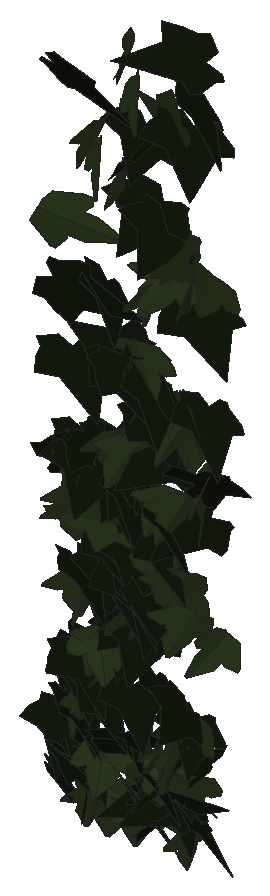
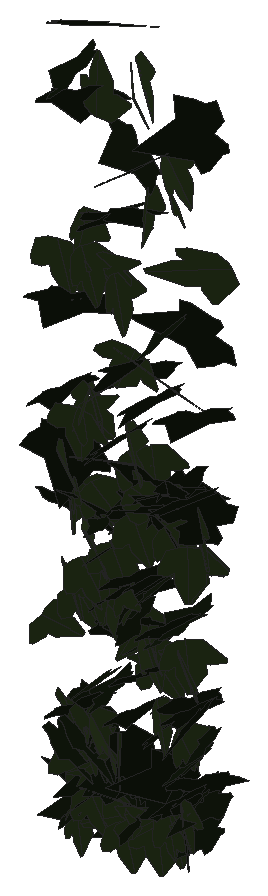
# SketchUp Ruby script. Lengths in inches.
U = 1.inch
M = Sketchup.active_model
def pt(a) = Geom::Point3d.new(a.map { |v| v * U })
def face(e, loops, mat)
  f = e.add_face(loops[0].map { |a| pt(a) })
  loops[1..].each { |l| e.add_face(l.map { |a| pt(a) }).erase! }
  f.material = f.back_material = mat if mat
  f
end
# faces: each face lists its corners as indices into pts; further lists are holes
def faces(e, pts, list, mat = nil) = list.each { |f| face(e, (f[0].is_a?(Array) ? f : [f]).map { |l| l.map { |i| pts[i] } }, mat) }
# xy, xz, yz: faces in a plane at the given z, y or x. An outline is a flat list of corners, or four numbers for a rectangle; further outlines are holes
def ring(l) = l.size == 4 ? [[l[0], l[1]], [l[2], l[1]], [l[2], l[3]], [l[0], l[3]]] : l.each_slice(2).to_a
def flat(e, list, mat, &to3) = list.each { |f| face(e, (f[0].is_a?(Array) ? f : [f]).map { |l| ring(l).map { |u, v| to3.(u, v) } }, mat) }
def xy(e, z, list, mat = nil) = flat(e, list, mat) { |x, y| [x, y, z] }
def xz(e, y, list, mat = nil) = flat(e, list, mat) { |x, z| [x, y, z] }
def yz(e, x, list, mat = nil) = flat(e, list, mat) { |y, z| [x, y, z] }
def lines(e, pts, list) = list.each { |a, b| e.add_line(pt(pts[a]), pt(pts[b])) }
# prism: a flat outline (further loops are holes) pulled along v
def prism(e, loops, v, mat = nil)
  f = face(e, loops, mat); d = Geom::Vector3d.new(v.map { |x| x * U })
  f.pushpull(f.normal.samedirection?(d) ? d.length : -d.length)
end
def box(e, o, s, mat = nil) = prism(e, [[o, [o[0] + s[0], o[1], o[2]], [o[0] + s[0], o[1] + s[1], o[2]], [o[0], o[1] + s[1], o[2]]]], [0, 0, s[2]], mat)
def at(x, y, z, deg = 0) = Geom::Transformation.translation(pt([x, y, z])) * Geom::Transformation.rotation(ORIGIN, Z_AXIS, deg.degrees)
def axes(o, x, y, z) = Geom::Transformation.new([*x, 0, *y, 0, *z, 0, *pt(o).to_a, 1])
def part(name) = M.definitions.add(name)
# library, detail: a bought-in or finely detailed component or shape, given as its bounding box
def library(name, o, s) = part(name).tap { |d| box(d.entities, o, s) }
def detail(e, o, s) = box(e.add_group.entities, o, s)
def put(e, d, t, mat = nil) = e.add_instance(d, t).tap { |i| i.material = mat if mat }
def group(e, t, mat = nil) = e.add_group.tap { |g| g.transformation = t; g.material = mat if mat }.entities
root = M.entities
M.materials.add("1026 AP 7946 SUNNY SIDE UP").color = [254, 231, 186]
M.materials.add("efeu1").color = [18, 25, 13]
M.materials.add("efeu2").color = [43, 57, 29]
c1 = part("ivyleaf_10")
p = [[0,0.5,-0.03],[-0.0625,2.02,-0.43],[-0.19,2.01,-0.46],[-0.54,1.05,-0.29],[-0.52,0.625,-0.18],[-0.83,0.76,-0.28],
  [-1.16,0.64,-0.33],[-1.15,0.33,-0.24],[-0.77,-0.39,0.02],[-0.3,-0.51,0.16],[0.04,-0.48,0.23],[-0.02,2.01,-0.4375],
  [-0.06,2.01,-0.43],[0.04,-0.49,0.23],[0.67,-0.49,0.14],[1.38,0.36,-0.2],[1.375,0.51,-0.24],[0.81,0.65,-0.19],
  [0.62,0.59,-0.15],[0.6,1.09,-0.28],[0.5,1.23,-0.31]]
faces(c1.entities,p,[[0,1,2,3,4,5,6,7,8,9,10],[11,12,0,13,14,15,16,17,18,19,20]],"efeu2")
c2 = part("ivyleaf_9")
p = [[1.54,2.16,1.25],[1.36,2.04,1.19],[-0.21,0.99,0.68],[-0.71,1.11,0.82],[-0.85,0.86,0.67],[-0.8,0.17,0.21],
  [-0.9,-0.01,0.1],[-0.67,-0.16,-0.02],[-0.08,-0.08,-0.05],[-0.03,-0.6,-0.4],[0.65,-0.88,-0.66],[0.83,-0.6,-0.49],
  [1.29,-0.42,-0.43],[1.8125,-0.07,-0.26],[1.21,0.44,0.15]]
faces(c2.entities,p,[[0,1,2,3,4,5,6,7,8,9,10,11,12,13,14]],"efeu1")
put(root,c1,axes([111.16,212.79,270.9],[-0.25846,-0.22574,0.01408],[0.03079,-0.0326,-0.2856],[0.3544,-0.1618,0.03508]),"1026 AP 7946 SUNNY SIDE UP")
put(root,c2,axes([111.02,212.73,270.01],[0.18307,-0.18563,-0.16634],[-0.13918,0.13382,-0.22493],[0.35979,0.14622,-0.00237]),"1026 AP 7946 SUNNY SIDE UP")
put(root,c2,axes([111.1,212.61,268.95],[-0.21823,-0.23774,-0.01451],[0.02596,0.00509,-0.28331],[0.37346,-0.13928,0.01122]),"1026 AP 7946 SUNNY SIDE UP")
put(root,c2,axes([111.03,212.36,268.65],[0.37718,-0.03348,-0.11398],[-0.14053,0.1073,-0.23284],[0.11482,0.2413,0.08945]),"1026 AP 7946 SUNNY SIDE UP")
put(root,c1,axes([111.21,212.71,272.2],[-0.28974,-0.20895,-0.01101],[0.02661,-0.00228,-0.28664],[0.32781,-0.18449,0.01354]),"1026 AP 7946 SUNNY SIDE UP")
put(root,c1,axes([111.15,212.85,270.75],[0.24057,-0.22294,0.04507],[0.03997,-0.03716,-0.27877],[0.35539,0.15509,0.00084]),"1026 AP 7946 SUNNY SIDE UP")
put(root,c2,axes([111.01,212.41,268.2],[0.32875,-0.14193,-0.07795],[-0.07623,0.06134,-0.25893],[0.24052,0.21343,0.02448]),"1026 AP 7946 SUNNY SIDE UP")
put(root,c1,axes([111.29,212.4375,272.7],[0.23704,-0.24789,-0.14116],[-0.07303,0.12988,-0.297],[0.43826,0.15572,0.02686]),"1026 AP 7946 SUNNY SIDE UP")
put(root,c1,axes([111.28,212.54,272.11],[-0.21849,-0.24101,-0.02736],[0.02828,0.0187,-0.28642],[0.37998,-0.13997,0.00559]),"1026 AP 7946 SUNNY SIDE UP")
put(root,c2,axes([110.98,212.5,272.71],[0.11914,0.00468,0.28145],[0.4221,0.05149,-0.07731],[-0.07996,0.27878,0.01124]),"1026 AP 7946 SUNNY SIDE UP")
put(root,c2,axes([111.15,212.62,274.31],[-0.07232,-0.26894,-0.11603],[0.07636,0.10381,-0.27897],[0.45113,-0.06068,0.02862]),"1026 AP 7946 SUNNY SIDE UP")
put(root,c2,axes([111.17,212.73,269.19],[0.05394,-0.25714,0.06466],[0.01516,-0.0635,-0.26762],[0.41647,0.03561,0.00137]),"1026 AP 7946 SUNNY SIDE UP")
put(root,c2,axes([111,212.51,278.44],[0.46882,-0.09984,0.08402],[0.11016,-0.04873,-0.32333],[0.17085,0.3054,-0.02209]),"1026 AP 7946 SUNNY SIDE UP")
put(root,c2,axes([111.16,212.46,269.32],[0.20675,-0.23514,0.01184],[-0.00657,-0.01702,-0.27737],[0.37023,0.13101,-0.01153]),"1026 AP 7946 SUNNY SIDE UP")
put(root,c1,axes([111.04,212.39,276.37],[-0.14408,-0.08172,-0.31235],[0.478,0.0542,-0.10955],[0.12093,-0.31162,0.06085]),"1026 AP 7946 SUNNY SIDE UP")
put(root,c2,axes([111.21,212.74,273.08],[0.01746,-0.27644,-0.08279],[0.03076,0.07939,-0.28366],[0.45094,0.00529,0.02255]),"1026 AP 7946 SUNNY SIDE UP")
put(root,c2,axes([111.23,212.34,268.62],[0.25425,-0.18608,-0.12792],[-0.11025,0.10197,-0.25304],[0.33307,0.1758,0.01389]),"1026 AP 7946 SUNNY SIDE UP")
put(root,c1,axes([111.41,212.79,272.52],[-0.18292,-0.21073,0.15461],[0.05122,-0.17635,-0.22829],[0.40466,-0.07293,0.09878]),"1026 AP 7946 SUNNY SIDE UP")
put(root,c1,axes([111.4375,212.57,268.41],[0.31397,-0.14487,-0.09904],[-0.06966,0.09792,-0.24836],[0.26363,0.19841,0.05232]),"1026 AP 7946 SUNNY SIDE UP")
put(root,c2,axes([111.3,212.55,269.875],[-0.02897,-0.26788,-0.02364],[0.00054,0.02146,-0.27649],[0.42255,-0.01839,-0.00127]),"1026 AP 7946 SUNNY SIDE UP")
put(root,c2,axes([111.6,212.33,268.21],[0.01774,-0.02013,-0.27651],[-0.37306,0.12588,-0.01928],[0.19948,0.2372,-0.01145]),"1026 AP 7946 SUNNY SIDE UP")
put(root,c1,axes([111.76,212.4,272.11],[0.11792,-0.02448,-0.28807],[-0.42407,0.07343,-0.08075],[0.12157,0.2799,-0.00225]),"1026 AP 7946 SUNNY SIDE UP")
put(root,c1,axes([111.44,212.51,269.39],[-0.03187,-0.24501,0.11408],[0.06089,-0.11393,-0.24991],[0.41929,-0.00208,0.04496]),"1026 AP 7946 SUNNY SIDE UP")
put(root,c2,axes([111.34,212.71,268.62],[0.01428,-0.26436,-0.03819],[-0.01447,0.03526,-0.27217],[0.41918,0.01022,-0.00809]),"1026 AP 7946 SUNNY SIDE UP")
put(root,c2,axes([111.33,212.53,270.02],[-0.01544,-0.26714,-0.10615],[0.01368,0.10126,-0.27476],[0.44916,-0.01227,0.00472]),"1026 AP 7946 SUNNY SIDE UP")
put(root,c2,axes([111.07,212.4,275.41],[0.17756,-0.03565,-0.29261],[0.36941,0.18565,0.07336],[0.25662,-0.24258,0.09686]),"1026 AP 7946 SUNNY SIDE UP")
put(root,c2,axes([111.3,212.58,271.2],[0.07275,-0.25296,0.09975],[0.07853,-0.09004,-0.26355],[0.41942,0.06074,0.03205]),"1026 AP 7946 SUNNY SIDE UP")
put(root,c2,axes([111.45,212.5,273.23],[0.09054,-0.1877,-0.21569],[-0.12355,0.19332,-0.20071],[0.42323,0.09659,-0.01245]),"1026 AP 7946 SUNNY SIDE UP")
put(root,c1,axes([111.625,212.51,268.09],[-0.15001,-0.26777,0.02721],[-0.00092,-0.02943,-0.29285],[0.42332,-0.09495,0.00901]),"1026 AP 7946 SUNNY SIDE UP")
put(root,c1,axes([111.62,212.51,277.78],[0.02832,-0.2977,0.06216],[-0.00462,-0.0623,-0.30754],[0.47813,0.01703,-0.00665]),"1026 AP 7946 SUNNY SIDE UP")
put(root,c2,axes([111.49,212.82,271.17],[-0.10353,-0.26958,0.02946],[0.00172,-0.03126,-0.28594],[0.42653,-0.06531,0.0083]),"1026 AP 7946 SUNNY SIDE UP")
put(root,c2,axes([111.58,212.53,272.95],[-0.27863,-0.23651,-0.01871],[0.02847,0.00744,-0.30423],[0.37173,-0.17784,0.00928]),"1026 AP 7946 SUNNY SIDE UP")
put(root,c1,axes([111.63,212.74,269.82],[0.03868,-0.2682,-0.04132],[0.01948,0.03982,-0.27675],[0.42562,0.02255,0.01642]),"1026 AP 7946 SUNNY SIDE UP")
put(root,c2,axes([111.46,212.9,271.85],[0.08262,-0.27136,0.03007],[-0.00016,-0.03131,-0.28486],[0.42941,0.0522,-0.00589]),"1026 AP 7946 SUNNY SIDE UP")
put(root,c1,axes([111.88,212.79,272.92],[-0.21743,-0.11557,0.22862],[-0.17064,-0.20156,-0.17845],[0.35551,-0.16743,0.05417]),"1026 AP 7946 SUNNY SIDE UP")
put(root,c1,axes([111.5625,212.58,277.39],[0.22743,-0.18145,0.19332],[0.2154,-0.13123,-0.23896],[0.35075,0.19825,0.0214]),"1026 AP 7946 SUNNY SIDE UP")
put(root,c2,axes([111.4375,212.48,268.71],[0.27503,0.06669,0.19674],[0.28969,0.0505,-0.19209],[-0.12996,0.25371,-0.01184]),"1026 AP 7946 SUNNY SIDE UP")
put(root,c1,axes([111.81,212.6,267.9],[-0.38126,-0.08092,0.04408],[-0.05632,-0.02903,-0.26299],[0.13282,-0.24458,0.01502]),"1026 AP 7946 SUNNY SIDE UP")
put(root,c2,axes([111.57,212.77,275.36],[0.04299,-0.27364,0.11977],[0.00071,-0.11827,-0.28379],[0.46845,0.02529,-0.01056]),"1026 AP 7946 SUNNY SIDE UP")
put(root,c1,axes([111.83,212.55,270.375],[-0.23292,-0.20064,0.1353],[-0.04028,-0.14155,-0.25118],[0.3759,-0.13949,0.05692]),"1026 AP 7946 SUNNY SIDE UP")
put(root,c2,axes([112.1,212.5,274.59],[-0.14094,0.20077,0.19345],[-0.27447,0.10961,-0.20718],[-0.33235,-0.17566,0.08906]),"1026 AP 7946 SUNNY SIDE UP")
put(root,c2,axes([111.62,212.53,269.56],[0.10649,-0.25155,-0.06729],[-0.02601,0.06171,-0.26801],[0.40726,0.06972,0.00048]),"1026 AP 7946 SUNNY SIDE UP")
put(root,c1,axes([111.76,212.46,268.68],[0.31294,0.17171,-0.04724],[-0.03914,-0.04271,-0.27055],[-0.2771,0.19994,-0.01514]),"1026 AP 7946 SUNNY SIDE UP")
put(root,c1,axes([111.875,212.68,270.65],[0.01039,-0.27822,0.0172],[-0.00063,-0.01829,-0.28681],[0.43842,0.00657,-0.00082]),"1026 AP 7946 SUNNY SIDE UP")
put(root,c1,axes([111.78,212.71,270.76],[0.18971,-0.23068,0.09571],[0.10543,-0.07076,-0.26736],[0.37736,0.13574,0.02658]),"1026 AP 7946 SUNNY SIDE UP")
put(root,c1,axes([111.74,212.41,270.37],[0.37299,0.1356,0.03339],[0.06446,-0.00827,-0.28012],[-0.20925,0.23917,-0.02677]),"1026 AP 7946 SUNNY SIDE UP")
put(root,c1,axes([111.92,212.52,273.36],[-0.15328,-0.26613,-0.02058],[0.01419,0.01635,-0.29187],[0.41923,-0.09786,0.00236]),"1026 AP 7946 SUNNY SIDE UP")
put(root,c1,axes([111.95,212.85,272.5],[-0.2289,-0.23113,0.07102],[-0.01115,-0.0779,-0.27962],[0.37968,-0.14163,0.03461]),"1026 AP 7946 SUNNY SIDE UP")
put(root,c2,axes([111.72,212.68,271.78],[0.02557,-0.28175,-0.04899],[0.01846,0.04665,-0.2901],[0.4485,0.01414,0.01474]),"1026 AP 7946 SUNNY SIDE UP")
put(root,c2,axes([111.9,212.87,272.74],[-0.2865,-0.21554,0.03044],[0.01372,-0.04732,-0.28853],[0.34208,-0.17862,0.03707]),"1026 AP 7946 SUNNY SIDE UP")
put(root,c2,axes([111.64,212.69,268.45],[0.0828,-0.16289,0.20919],[0.15416,-0.18052,-0.17564],[0.38042,0.10861,0.02564]),"1026 AP 7946 SUNNY SIDE UP")
put(root,c2,axes([111.87,212.92,270.37],[-0.15472,-0.24477,0.06216],[0.00463,-0.06736,-0.27073],[0.3969,-0.09463,0.02739]),"1026 AP 7946 SUNNY SIDE UP")
put(root,c2,axes([111.73,212.79,273.23],[-0.16285,-0.16476,-0.21714],[0.32064,0.09627,-0.18099],[0.27052,-0.21329,0.0838]),"1026 AP 7946 SUNNY SIDE UP")
put(root,c2,axes([111.77,212.7,274.375],[0.07629,-0.27385,-0.10286],[0.00648,0.10028,-0.28516],[0.45745,0.04425,0.02119]),"1026 AP 7946 SUNNY SIDE UP")
put(root,c2,axes([111.85,212.76,272.67],[-0.25159,-0.07127,-0.22509],[0.35615,-0.00667,-0.16899],[0.05752,-0.2704,0.0618]),"1026 AP 7946 SUNNY SIDE UP")
put(root,c1,axes([111.97,212.53,277.15],[0.07505,-0.27677,-0.10696],[0.07507,0.10947,-0.28163],[0.45784,0.02742,0.06371]),"1026 AP 7946 SUNNY SIDE UP")
put(root,c2,axes([111.98,212.84,272.81],[-0.21624,-0.24121,0.06611],[-0.01669,-0.0691,-0.28534],[0.39267,-0.13577,0.02427]),"1026 AP 7946 SUNNY SIDE UP")
put(root,c1,axes([112.05,212.6,279.05],[0.1584,-0.28964,-0.0546],[-0.01324,0.05143,-0.31549],[0.46234,0.1007,0.00968]),"1026 AP 7946 SUNNY SIDE UP")
put(root,c2,axes([111.98,212.6875,270.64],[-0.20538,-0.17712,0.17917],[0.00019,-0.19758,-0.20717],[0.39143,-0.09284,0.09411]),"1026 AP 7946 SUNNY SIDE UP")
put(root,c1,axes([112.09,212.76,273.71],[0.11088,-0.27678,-0.06673],[-0.02168,0.06171,-0.29387],[0.44588,0.07183,0.00231]),"1026 AP 7946 SUNNY SIDE UP")
put(root,c1,axes([112.16,212.59,273.24],[-0.18839,-0.21685,0.16013],[-0.035,-0.16298,-0.25089],[0.41919,-0.11106,0.05102]),"1026 AP 7946 SUNNY SIDE UP")
put(root,c1,axes([111.91,212.61,268.06],[0.15644,0.14512,0.20508],[0.15592,0.17196,-0.17995],[-0.35344,0.1401,0.01139]),"1026 AP 7946 SUNNY SIDE UP")
put(root,c2,axes([112.02,212.43,268.98],[0.30608,0.18291,0.02594],[0.05096,0.00064,-0.27426],[-0.28559,0.19615,-0.02114]),"1026 AP 7946 SUNNY SIDE UP")
put(root,c2,axes([112.04,212.98,277.7],[-0.13932,-0.26153,0.11927],[0.00228,-0.12315,-0.28253],[0.45067,-0.08023,0.0383]),"1026 AP 7946 SUNNY SIDE UP")
put(root,c1,axes([112.18,212.76,267.87],[-0.2446,-0.20952,0.03719],[0.00438,-0.0482,-0.26725],[0.3346,-0.15253,0.03069]),"1026 AP 7946 SUNNY SIDE UP")
put(root,c2,axes([112.07,212.8,271.69],[-0.13197,-0.26759,0.01194],[0.00912,-0.01555,-0.28881],[0.42117,-0.08351,0.00999]),"1026 AP 7946 SUNNY SIDE UP")
put(root,c2,axes([112.03,212.73,272.55],[-0.02936,-0.26574,0.11334],[0.01683,-0.11232,-0.27453],[0.45285,-0.01305,0.01755]),"1026 AP 7946 SUNNY SIDE UP")
put(root,c1,axes([112.16,212.39,270.87],[-0.10633,-0.21266,-0.22532],[0.14199,0.19874,-0.22793],[0.45676,-0.11129,0.01841]),"1026 AP 7946 SUNNY SIDE UP")
put(root,c2,axes([112.1,212.55,271.42],[-0.08499,-0.26836,-0.06513],[0.02002,0.06038,-0.28166],[0.43252,-0.05553,0.00024]),"1026 AP 7946 SUNNY SIDE UP")
put(root,c2,axes([112.09,212.67,269.67],[-0.03683,-0.2761,-0.01817],[0.00797,0.0157,-0.28534],[0.4348,-0.02367,0.00369]),"1026 AP 7946 SUNNY SIDE UP")
put(root,c2,axes([111.97,212.79,271.09],[0.2428,-0.21898,0.07818],[0.06371,-0.06579,-0.27639],[0.35946,0.15958,-0.00382]),"1026 AP 7946 SUNNY SIDE UP")
put(root,c2,axes([112.07,212.72,268.12],[0.28372,-0.19281,-0.00282],[-0.02004,-0.00969,-0.2716],[0.30252,0.18018,-0.01535]),"1026 AP 7946 SUNNY SIDE UP")
put(root,c1,axes([112.39,212.75,271.9],[-0.30448,-0.18758,0.08222],[-0.01057,-0.10552,-0.26935],[0.32103,-0.18139,0.06911]),"1026 AP 7946 SUNNY SIDE UP")
put(root,c2,axes([112.38,212.3,277.67],[-0.21295,0.20476,-0.20307],[-0.14326,0.17691,0.25335],[0.42467,0.16236,-0.01636]),"1026 AP 7946 SUNNY SIDE UP")
put(root,c1,axes([112.35,212.66,269.04],[0.09195,-0.25133,-0.08147],[0.03376,0.08385,-0.26241],[0.41224,0.04919,0.03966]),"1026 AP 7946 SUNNY SIDE UP")
put(root,c2,axes([112.125,212.57,271.18],[0.12771,-0.24366,0.10852],[0.04541,-0.10285,-0.26516],[0.41581,0.08607,-0.00438]),"1026 AP 7946 SUNNY SIDE UP")
put(root,c2,axes([112.12,212.45,274.61],[0.06742,-0.239,-0.19751],[0.09943,0.19501,-0.23641],[0.47004,-0.00697,0.07834]),"1026 AP 7946 SUNNY SIDE UP")
put(root,c1,axes([112.31,212.54,274.7],[-0.42802,0.04324,-0.08897],[0.10282,-0.10846,-0.26814],[-0.11224,-0.26426,0.09365]),"1026 AP 7946 SUNNY SIDE UP")
put(root,c2,axes([112.59,212.74,268.26],[-0.41159,-0.00773,0.04508],[-0.05948,-0.09892,-0.25141],[0.0368,-0.24628,0.09789]),"1026 AP 7946 SUNNY SIDE UP")
put(root,c1,axes([112.4,212.68,271],[0.02898,-0.21953,0.1827],[0.03802,-0.1771,-0.22787],[0.44336,0.02954,0.0076]),"1026 AP 7946 SUNNY SIDE UP")
put(root,c2,axes([112.2,212.77,273.71],[0.1302,-0.26337,-0.10162],[-0.01055,0.0994,-0.28292],[0.44127,0.08009,0.02322]),"1026 AP 7946 SUNNY SIDE UP")
put(root,c1,axes([112.19,212.54,278.56],[0.19897,-0.11768,0.25994],[0.27844,-0.1808,-0.17895],[0.33905,0.21754,-0.00558]),"1026 AP 7946 SUNNY SIDE UP")
put(root,c2,axes([112.47,212.74,276.87],[-0.33655,-0.20901,0.05606],[-0.01009,-0.07205,-0.30491],[0.33993,-0.20908,0.04645]),"1026 AP 7946 SUNNY SIDE UP")
put(root,c2,axes([112.42,212.54,270.75],[-0.25067,-0.22647,-0.01409],[0.02292,0.00488,-0.28513],[0.3559,-0.15983,0.00844]),"1026 AP 7946 SUNNY SIDE UP")
put(root,c1,axes([112.48,212.55,275.69],[-0.02663,-0.29967,-0.02807],[0.02088,0.02482,-0.30882],[0.47244,-0.01799,0.01206]),"1026 AP 7946 SUNNY SIDE UP")
put(root,c2,axes([112.71,212.39,268.55],[-0.19917,0.24624,0.00136],[-0.01589,-0.00528,-0.28506],[-0.38686,-0.12656,0.011]),"1026 AP 7946 SUNNY SIDE UP")
put(root,c1,axes([112.54,212.54,268.84],[0.0918,-0.26057,0.00276],[-0.00584,-0.00509,-0.27508],[0.40973,0.05831,-0.00454]),"1026 AP 7946 SUNNY SIDE UP")
put(root,c2,axes([112.63,212.8,273.21],[-0.39722,-0.11769,0.06822],[-0.01035,-0.13078,-0.26341],[0.21261,-0.22625,0.11464]),"1026 AP 7946 SUNNY SIDE UP")
put(root,c1,axes([112.57,212.65,271.33],[-0.43709,0.02439,0.00365],[-0.00896,-0.02615,-0.28632],[-0.03768,-0.27676,0.02572]),"1026 AP 7946 SUNNY SIDE UP")
put(root,c1,axes([112.26,212.77,268.1],[0.25938,0.00426,0.21259],[0.31762,0.05079,-0.16715],[-0.06649,0.25924,0.03083]),"1026 AP 7946 SUNNY SIDE UP")
put(root,c1,axes([112.66,212.84,268.23],[-0.23368,-0.19882,0.08029],[-0.03773,-0.08017,-0.25463],[0.33432,-0.14802,0.02738]),"1026 AP 7946 SUNNY SIDE UP")
put(root,c2,axes([112.4,212.71,272],[0.10165,-0.2757,-0.05196],[-0.00487,0.04945,-0.29132],[0.44024,0.06421,0.00877]),"1026 AP 7946 SUNNY SIDE UP")
put(root,c1,axes([112.61,212.8,269.3125],[0.07654,-0.25801,0.07112],[0.00557,-0.07103,-0.27074],[0.42054,0.0479,-0.00936]),"1026 AP 7946 SUNNY SIDE UP")
put(root,c2,axes([112.52,212.5625,271.14],[-0.1012,-0.2547,0.08217],[-0.0144,-0.08138,-0.27089],[0.4201,-0.06414,0.01051]),"1026 AP 7946 SUNNY SIDE UP")
put(root,c2,axes([112.4,212.76,269.87],[0.1175,-0.25054,0.08571],[0.02811,-0.08295,-0.26974],[0.41486,0.07658,-0.006]),"1026 AP 7946 SUNNY SIDE UP")
put(root,c1,axes([112.7,212.67,272.65],[-0.19321,-0.20645,0.15044],[-0.03457,-0.15429,-0.24273],[0.39719,-0.11386,0.05206]),"1026 AP 7946 SUNNY SIDE UP")
put(root,c1,axes([112.48,212.54,268.72],[-0.27395,-0.11486,-0.18432],[0.24925,0.08272,-0.21402],[0.22151,-0.23513,0.01287]),"1026 AP 7946 SUNNY SIDE UP")
put(root,c2,axes([112.78,212.35,268.12],[-0.06247,0.25659,-0.04617],[0.0085,-0.04599,-0.26775],[-0.40988,-0.04006,0.00149]),"1026 AP 7946 SUNNY SIDE UP")
put(root,c2,axes([112.52,212.57,274.28],[-0.01948,-0.28299,0.08559],[-0.00246,-0.08469,-0.2923],[0.46446,-0.01232,0.00204]),"1026 AP 7946 SUNNY SIDE UP")
put(root,c2,axes([112.42,212.74,268.65],[0.38756,-0.10381,0.00553],[0.01637,0.00938,-0.27515],[0.16267,0.24637,0.01451]),"1026 AP 7946 SUNNY SIDE UP")
put(root,c1,axes([112.79,212.63,275.92],[-0.30208,-0.14315,0.18906],[-0.08249,-0.20616,-0.22246],[0.35759,-0.16848,0.1084]),"1026 AP 7946 SUNNY SIDE UP")
put(root,c2,axes([112.44,212.55,268.68],[0.14806,-0.22706,0.09909],[0.05864,-0.09006,-0.25376],[0.38408,0.10128,0.00054]),"1026 AP 7946 SUNNY SIDE UP")
put(root,c2,axes([112.68,212.625,276.66],[-0.1948,-0.24872,0.12763],[-0.03956,-0.12658,-0.28522],[0.43613,-0.12257,0.03113]),"1026 AP 7946 SUNNY SIDE UP")
put(root,c2,axes([112.82,212.61,268.29],[-0.28976,-0.12015,0.13891],[-0.112,-0.12968,-0.21898],[0.26184,-0.18843,0.06005]),"1026 AP 7946 SUNNY SIDE UP")
put(root,c1,axes([112.85,212.72,271.49],[-0.25267,-0.2175,0.09541],[-0.06322,-0.08671,-0.27846],[0.36707,-0.16465,0.01772]),"1026 AP 7946 SUNNY SIDE UP")
put(root,c1,axes([112.8,212.8,276.1],[-0.08157,-0.29749,0.01521],[0.00473,-0.01723,-0.31114],[0.46847,-0.05162,0.00579]),"1026 AP 7946 SUNNY SIDE UP")
put(root,c2,axes([112.53,212.66,272.38],[0.13256,-0.25287,0.11369],[0.05775,-0.1056,-0.27521],[0.43088,0.09195,0.00191]),"1026 AP 7946 SUNNY SIDE UP")
put(root,c1,axes([112.8,212.64,273.99],[0.18198,-0.25357,-0.0795],[-0.02897,0.07474,-0.28636],[0.41511,0.11638,0.01487]),"1026 AP 7946 SUNNY SIDE UP")
put(root,c1,axes([112.59,212.48,268.64],[0.06307,-0.08879,-0.25623],[0.27806,0.19527,-0.04138],[0.30742,-0.1584,0.08999]),"1026 AP 7946 SUNNY SIDE UP")
put(root,c2,axes([112.43,212.59,268.2],[0.3005,0.08651,-0.18215],[0.22195,0.11249,0.21395],[0.21671,-0.23517,0.03346]),"1026 AP 7946 SUNNY SIDE UP")
put(root,c1,axes([112.86,212.66,272.61],[-0.15007,-0.22935,0.14133],[-0.01306,-0.14441,-0.25312],[0.42108,-0.08622,0.04252]),"1026 AP 7946 SUNNY SIDE UP")
put(root,c1,axes([112.81,212.72,271.95],[0.24137,-0.23323,0.03149],[0.00846,-0.03459,-0.28746],[0.37005,0.15292,-0.01397]),"1026 AP 7946 SUNNY SIDE UP")
put(root,c1,axes([112.84,212.72,273.77],[-0.08048,-0.2105,0.20439],[0.0412,-0.2052,-0.21723],[0.45426,-0.01868,0.05591]),"1026 AP 7946 SUNNY SIDE UP")
put(root,c1,axes([112.77,212.62,268.84],[0.02643,-0.20079,0.18148],[0.11289,-0.16778,-0.20373],[0.40579,0.05975,0.04486]),"1026 AP 7946 SUNNY SIDE UP")
put(root,c2,axes([113.03,212.72,269.1],[-0.21066,0.2229,-0.01347],[-0.00367,-0.01812,-0.26777],[-0.3512,-0.13351,0.01088]),"1026 AP 7946 SUNNY SIDE UP")
put(root,c1,axes([112.87,212.46,269.09],[0.15175,-0.25395,0.01808],[-0.00184,-0.02075,-0.27986],[0.40042,0.09615,-0.00814]),"1026 AP 7946 SUNNY SIDE UP")
put(root,c2,axes([112.72,212.85,268.23],[0.02359,-0.26147,0.03424],[-0.01007,-0.03513,-0.26988],[0.41463,0.01402,-0.00851]),"1026 AP 7946 SUNNY SIDE UP")
put(root,c1,axes([112.85,212.48,278.23],[-0.4422,0.13443,0.0676],[0.10176,-0.01485,0.3207],[0.21148,0.28823,-0.01295]),"1026 AP 7946 SUNNY SIDE UP")
put(root,c1,axes([112.99,212.77,273.67],[-0.43584,0.06512,0.02566],[-0.06361,-0.06877,-0.28311],[-0.08904,-0.26963,0.07663]),"1026 AP 7946 SUNNY SIDE UP")
put(root,c1,axes([113.03,212.64,271.01],[-0.25664,-0.18927,0.12388],[-0.04324,-0.132,-0.25101],[0.35085,-0.15471,0.05968]),"1026 AP 7946 SUNNY SIDE UP")
put(root,c1,axes([112.92,212.74,274.02],[-0.23196,0.24324,-0.02491],[0.00144,-0.0293,-0.29287],[-0.38458,-0.14682,0.01393]),"1026 AP 7946 SUNNY SIDE UP")
put(root,c1,axes([112.98,212.73,267.82],[-0.0654,-0.2599,-0.0033],[0.04818,-0.00317,-0.26932],[0.40583,-0.04151,0.03144]),"1026 AP 7946 SUNNY SIDE UP")
put(root,c2,axes([112.9375,212.65,269.65],[-0.13553,-0.18425,0.18295],[-0.03863,-0.18165,-0.20629],[0.40167,-0.07964,0.04189]),"1026 AP 7946 SUNNY SIDE UP")
put(root,c1,axes([112.91,212.57,269.1],[0.06787,-0.15986,0.22921],[0.12652,-0.20886,-0.17121],[0.413,0.09026,0.01478]),"1026 AP 7946 SUNNY SIDE UP")
put(root,c2,axes([113.07,212.2,269.15],[0.04857,0.23689,0.14575],[0.03395,0.13849,-0.24528],[-0.43145,0.03757,-0.00289]),"1026 AP 7946 SUNNY SIDE UP")
put(root,c1,axes([113.05,212.67,268.61],[-0.30823,-0.1699,0.01579],[0.00056,-0.02522,-0.26665],[0.26838,-0.19508,0.0187]),"1026 AP 7946 SUNNY SIDE UP")
put(root,c2,axes([113.3,212.5625,279.3],[-0.39697,0.00575,0.18144],[-0.23935,-0.16203,-0.22033],[0.13948,-0.2617,0.13828]),"1026 AP 7946 SUNNY SIDE UP")
put(root,c2,axes([113.21,212.8,272.47],[-0.44212,-0.05122,-0.00164],[0.01053,-0.02954,-0.29295],[0.07987,-0.27962,0.02954]),"1026 AP 7946 SUNNY SIDE UP")
put(root,c1,axes([113.05,212.48,276.42],[-0.04165,-0.27644,-0.15728],[0.08405,0.14549,-0.28302],[0.48819,-0.04863,0.03531]),"1026 AP 7946 SUNNY SIDE UP")
put(root,c2,axes([113.01,212.78,269.48],[-0.11514,-0.26015,0.03481],[-0.00426,-0.03586,-0.27853],[0.41278,-0.07293,0.00684]),"1026 AP 7946 SUNNY SIDE UP")
put(root,c2,axes([113.29,212.72,268.93],[-0.22263,0.21707,-0.05285],[0.02231,-0.05333,-0.26673],[-0.35047,-0.14129,0.01659]),"1026 AP 7946 SUNNY SIDE UP")
put(root,c1,axes([113.15,212.6875,272.61],[0.21754,-0.21493,-0.13587],[-0.02476,0.14143,-0.25601],[0.39473,0.12732,0.05882]),"1026 AP 7946 SUNNY SIDE UP")
put(root,c1,axes([113.16,212.46,276],[0.11211,-0.25945,-0.14736],[-0.00551,0.14488,-0.27451],[0.46471,0.06431,0.0323]),"1026 AP 7946 SUNNY SIDE UP")
put(root,c2,axes([112.92,212.81,268.07],[0.23436,-0.21601,0.02473],[0.01844,-0.02256,-0.27048],[0.34147,0.14947,-0.00237]),"1026 AP 7946 SUNNY SIDE UP")
put(root,c1,axes([113.12,212.71,269.38],[0.36061,-0.14498,0.00578],[0.00823,-0.00376,-0.27954],[0.22805,0.2294,0.00095]),"1026 AP 7946 SUNNY SIDE UP")
put(root,c1,axes([113.15,212.82,273.05],[0.21511,-0.24058,0.08044],[0.03956,-0.07695,-0.28511],[0.39642,0.13823,-0.0152]),"1026 AP 7946 SUNNY SIDE UP")
put(root,c1,axes([113.34,212.72,276],[-0.42634,0.0568,0.10226],[-0.16707,-0.03283,-0.28075],[-0.06532,-0.28675,0.05063]),"1026 AP 7946 SUNNY SIDE UP")
put(root,c2,axes([113.19,212.59,273.18],[0.33119,0.16209,-0.10467],[-0.122,-0.06725,-0.27413],[-0.2758,0.22439,-0.00443]),"1026 AP 7946 SUNNY SIDE UP")
put(root,c1,axes([113.24,212.61,271.25],[0.25574,-0.21265,-0.07563],[-0.0482,0.0673,-0.27491],[0.34981,0.16473,0.01742]),"1026 AP 7946 SUNNY SIDE UP")
put(root,c2,axes([113.05,212.81,275.48],[-0.14282,-0.22182,-0.17405],[0.13756,0.14466,-0.2451],[0.41504,-0.12428,0.02134]),"1026 AP 7946 SUNNY SIDE UP")
put(root,c2,axes([113.17,212.52,278.3],[-0.22292,-0.26542,-0.07446],[0.06373,0.05855,-0.30955],[0.4272,-0.14723,0.00733]),"1026 AP 7946 SUNNY SIDE UP")
put(root,c1,axes([113.36,212.88,270.67],[0.13213,0.16567,-0.22092],[-0.18705,-0.18027,-0.19171],[-0.38415,0.14476,0.01737]),"1026 AP 7946 SUNNY SIDE UP")
put(root,c2,axes([113.21,212.81,274.07],[-0.04498,-0.2913,-0.02487],[-0.00581,0.02295,-0.30134],[0.45937,-0.02824,-0.00625]),"1026 AP 7946 SUNNY SIDE UP")
put(root,c2,axes([113.12,212.65,278.66],[0.13297,-0.28211,0.10442],[0.02765,-0.10213,-0.30376],[0.4714,0.08557,-0.01163]),"1026 AP 7946 SUNNY SIDE UP")
